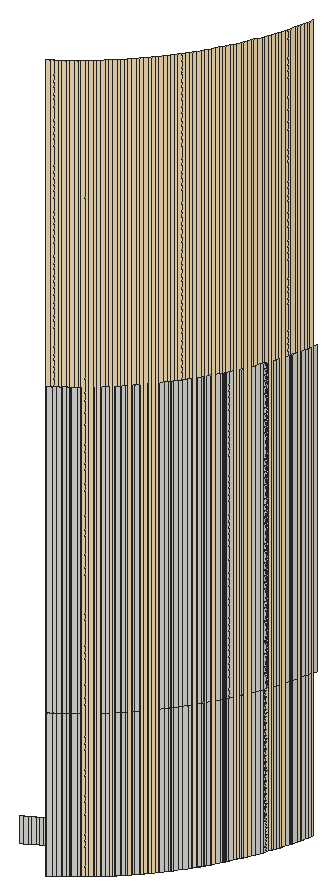
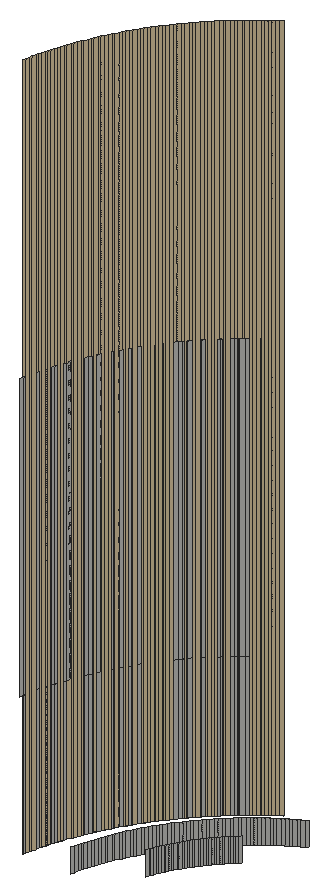
# SketchUp Ruby script. Lengths in inches.
U = 1.inch
M = Sketchup.active_model
def pt(a) = Geom::Point3d.new(a.map { |v| v * U })
def face(e, loops, mat)
  f = e.add_face(loops[0].map { |a| pt(a) })
  loops[1..].each { |l| e.add_face(l.map { |a| pt(a) }).erase! }
  f.material = f.back_material = mat if mat
  f
end
# faces: each face lists its corners as indices into pts; further lists are holes
def faces(e, pts, list, mat = nil) = list.each { |f| face(e, (f[0].is_a?(Array) ? f : [f]).map { |l| l.map { |i| pts[i] } }, mat) }
# xy, xz, yz: faces in a plane at the given z, y or x. An outline is a flat list of corners, or four numbers for a rectangle; further outlines are holes
def ring(l) = l.size == 4 ? [[l[0], l[1]], [l[2], l[1]], [l[2], l[3]], [l[0], l[3]]] : l.each_slice(2).to_a
def flat(e, list, mat, &to3) = list.each { |f| face(e, (f[0].is_a?(Array) ? f : [f]).map { |l| ring(l).map { |u, v| to3.(u, v) } }, mat) }
def xy(e, z, list, mat = nil) = flat(e, list, mat) { |x, y| [x, y, z] }
def xz(e, y, list, mat = nil) = flat(e, list, mat) { |x, z| [x, y, z] }
def yz(e, x, list, mat = nil) = flat(e, list, mat) { |y, z| [x, y, z] }
def lines(e, pts, list) = list.each { |a, b| e.add_line(pt(pts[a]), pt(pts[b])) }
# prism: a flat outline (further loops are holes) pulled along v
def prism(e, loops, v, mat = nil)
  f = face(e, loops, mat); d = Geom::Vector3d.new(v.map { |x| x * U })
  f.pushpull(f.normal.samedirection?(d) ? d.length : -d.length)
end
def box(e, o, s, mat = nil) = prism(e, [[o, [o[0] + s[0], o[1], o[2]], [o[0] + s[0], o[1] + s[1], o[2]], [o[0], o[1] + s[1], o[2]]]], [0, 0, s[2]], mat)
def at(x, y, z, deg = 0) = Geom::Transformation.translation(pt([x, y, z])) * Geom::Transformation.rotation(ORIGIN, Z_AXIS, deg.degrees)
def axes(o, x, y, z) = Geom::Transformation.new([*x, 0, *y, 0, *z, 0, *pt(o).to_a, 1])
def part(name) = M.definitions.add(name)
# library, detail: a bought-in or finely detailed component or shape, given as its bounding box
def library(name, o, s) = part(name).tap { |d| box(d.entities, o, s) }
def detail(e, o, s) = box(e.add_group.entities, o, s)
def put(e, d, t, mat = nil) = e.add_instance(d, t).tap { |i| i.material = mat if mat }
def group(e, t, mat = nil) = e.add_group.tap { |g| g.transformation = t; g.material = mat if mat }.entities
root = M.entities
M.materials.add("1026 AP 7946 SUNNY SIDE UP").color = [254, 231, 186]
p = [[183.75,229.08,246],[183.64,229,246],[183.64,229,276],[183.75,229.08,276],[183.8,229.11,252],[183.67,229.02,252],
  [183.67,229.02,246],[183.8,229.11,246],[183.85,229.15,246],[183.85,229.15,276],[183.95,229.22,246],[183.95,229.22,276],
  [183.93,229.2,252],[183.93,229.2,246],[184.05,229.29,252],[184.05,229.29,246],[184.05,229.29,246],[184.05,229.29,276],
  [184.15,229.37,246],[184.15,229.37,276],[184.18,229.38,252],[184.18,229.38,246],[184.26,229.44,246],[184.26,229.44,276],
  [184.31,229.48,252],[184.31,229.48,246],[184.35,229.52,246],[184.35,229.52,276],[184.43,229.58,252],[184.43,229.58,246],
  [184.45,229.6,246],[184.45,229.6,276],[184.55,229.67,252],[184.55,229.67,246],[184.55,229.67,246],[184.55,229.67,276],
  [184.65,229.75,246],[184.65,229.75,276],[184.67,229.77,252],[184.67,229.77,246],[184.75,229.83,246],[184.75,229.83,276],
  [184.84,229.92,246],[184.84,229.92,276],[184.79,229.875,252],[184.79,229.875,246],[184.9375,230,246],[184.9375,230,276],
  [184.91,229.98,252],[184.91,229.98,246],[185.03,230.08,246],[185.03,230.08,276],[185.03,230.08,252],[185.03,230.08,246],
  [185.12,230.17,246],[185.12,230.17,276],[185.15,230.1875,252],[185.15,230.1875,246],[181.77,230.21,246],[181.66,230.15,246],
  [181.66,230.15,247],[181.77,230.21,247],[181.89,230.28,246],[181.89,230.28,247],[185.21,230.25,246],[185.21,230.25,276],
  [185.26,230.3,252],[185.26,230.3,246],[182,230.34,246],[182,230.34,247],[182.11,230.41,246],[182.11,230.41,247],
  [185.31,230.34,246],[185.31,230.34,276],[185.4,230.43,246],[185.4,230.43,276],[185.375,230.4,252],[185.375,230.4,246],
  [182.22,230.47,246],[182.22,230.47,247],[185.49,230.51,246],[185.49,230.51,276],[185.49,230.51,252],[185.49,230.51,246],
  [182.34,230.54,246],[182.34,230.54,247],[182.45,230.61,246],[182.45,230.61,247],[185.57,230.6,246],[185.57,230.6,276],
  [185.6,230.625,252],[185.6,230.625,246],[182.56,230.69,246],[182.56,230.69,247],[185.66,230.69,246],[185.66,230.69,276],
  [185.7,230.74,252],[185.7,230.74,246],[182.66,230.76,246],[182.66,230.76,247],[185.75,230.79,246],[185.75,230.79,276],
  [185.8125,230.85,252],[185.8125,230.85,246],[182.77,230.83,246],[182.77,230.83,247],[182.88,230.91,246],[182.88,230.91,247],
  [185.83,230.88,246],[185.83,230.88,276],[182.98,230.99,246],[182.98,230.99,247],[185.92,230.97,246],[185.92,230.97,276],
  [185.92,230.97,252],[185.92,230.97,246],[183.09,231.07,246],[183.09,231.07,247],[186,231.0625,246],[186,231.0625,276],
  [186.02,231.09,252],[186.02,231.09,246],[183.19,231.15,246],[183.19,231.15,247],[183.29,231.23,246],[183.29,231.23,247],
  [186.08,231.16,246],[186.08,231.16,276],[186.125,231.21,252],[186.125,231.21,246],[183.39,231.3125,246],[183.39,231.3125,247],
  [186.17,231.25,246],[186.17,231.25,276],[186.23,231.33,252],[186.23,231.33,246],[183.49,231.4,246],[183.49,231.4,247],
  [186.25,231.35,246],[186.25,231.35,276],[186.33,231.45,252],[186.33,231.45,246],[183.59,231.48,246],[183.59,231.48,247],
  [186.33,231.45,246],[186.33,231.45,276],[186.4,231.55,246],[186.4,231.55,276],[186.42,231.57,252],[186.42,231.57,246],
  [183.69,231.57,246],[183.69,231.57,247],[186.48,231.65,246],[186.48,231.65,276],[183.79,231.66,246],[183.79,231.66,247],
  [186.52,231.69,252],[186.52,231.69,246],[186.56,231.74,246],[186.56,231.74,276],[183.88,231.75,246],[183.88,231.75,247],
  [183.98,231.84,246],[183.98,231.84,247],[186.62,231.82,252],[186.62,231.82,246],[186.63,231.85,246],[186.63,231.85,276],
  [184.07,231.93,246],[184.07,231.93,247],[186.71,231.95,246],[186.71,231.95,276],[186.71,231.95,252],[186.71,231.95,246],
  [184.16,232.02,246],[184.16,232.02,247],[186.78,232.05,246],[186.78,232.05,276],[186.8,232.07,252],[186.8,232.07,246],
  [184.25,232.12,246],[184.25,232.12,247],[186.85,232.15,246],[186.85,232.15,276],[184.34,232.21,246],[184.34,232.21,247],
  [186.89,232.2,252],[186.89,232.2,246],[184.43,232.31,246],[184.43,232.31,247],[186.92,232.25,246],[186.92,232.25,276],
  [186.98,232.33,252],[186.98,232.33,246],[184.52,232.41,246],[184.52,232.41,247],[187,232.36,246],[187,232.36,276],
  [187.0625,232.46,252],[187.0625,232.46,246],[184.6,232.51,246],[184.6,232.51,247],[187.0625,232.46,246],[187.0625,232.46,276],
  [184.6875,232.61,246],[184.6875,232.61,247],[187.13,232.57,246],[187.13,232.57,276],[187.15,232.6,252],[187.15,232.6,246],
  [184.77,232.71,246],[184.77,232.71,247],[187.2,232.68,246],[187.2,232.68,276],[187.23,232.73,252],[187.23,232.73,246],
  [184.85,232.81,246],[184.85,232.81,247],[187.26,232.78,246],[187.26,232.78,276],[187.3125,232.86,252],[187.3125,232.86,246],
  [184.93,232.91,246],[184.93,232.91,247],[187.33,232.89,246],[187.33,232.89,276],[185.01,233.02,246],[185.01,233.02,247],
  [187.39,233,246],[187.39,233,276],[187.39,233,252],[187.39,233,246],[185.09,233.12,246],[185.09,233.12,247],
  [187.45,233.11,246],[187.45,233.11,276],[187.47,233.14,252],[187.47,233.14,246],[185.17,233.23,246],[185.17,233.23,247],
  [187.52,233.22,246],[187.52,233.22,276],[187.55,233.27,252],[187.55,233.27,246],[185.24,233.34,246],[185.24,233.34,247],
  [187.58,233.33,246],[187.58,233.33,276],[185.31,233.44,246],[185.31,233.44,247],[187.62,233.41,252],[187.62,233.41,246],
  [187.63,233.44,246],[187.63,233.44,276],[185.39,233.55,246],[185.39,233.55,247],[187.69,233.55,246],[187.69,233.55,276],
  [187.69,233.55,252],[187.69,233.55,246],[185.46,233.66,246],[185.46,233.66,247],[187.75,233.66,246],[187.75,233.66,276],
  [187.76,233.69,252],[187.76,233.69,246],[185.53,233.78,246],[185.53,233.78,247],[187.8,233.78,246],[187.8,233.78,276],
  [187.83,233.83,252],[187.83,233.83,246],[185.59,233.89,246],[185.59,233.89,247],[187.86,233.89,246],[187.86,233.89,276],
  [187.9,233.98,252],[187.9,233.98,246],[185.66,234,246],[185.66,234,247],[187.91,234,246],[187.91,234,276],
  [185.72,234.11,246],[185.72,234.11,247],[187.96,234.12,246],[187.96,234.12,276],[187.96,234.12,252],[187.96,234.12,246],
  [185.79,234.23,246],[185.79,234.23,247],[188.01,234.23,246],[188.01,234.23,276],[188.03,234.26,252],[188.03,234.26,246],
  [185.85,234.34,246],[185.85,234.34,247],[188.0625,234.35,246],[188.0625,234.35,276],[185.91,234.46,246],[185.91,234.46,247],
  [188.09,234.41,252],[188.09,234.41,246],[188.11,234.47,246],[188.11,234.47,276],[188.15,234.55,252],[188.15,234.55,246],
  [185.97,234.58,246],[185.97,234.58,247],[188.16,234.58,246],[188.16,234.58,276],[186.03,234.69,246],[186.03,234.69,247],
  [188.2,234.7,252],[188.2,234.7,246],[188.2,234.7,246],[188.2,234.7,276],[186.08,234.8125,246],[186.08,234.8125,247],
  [188.25,234.82,246],[188.25,234.82,276],[188.26,234.85,252],[188.26,234.85,246],[186.14,234.93,246],[186.14,234.93,247],
  [188.29,234.94,246],[188.29,234.94,276],[188.3125,234.99,252],[188.3125,234.99,246],[186.1875,235.05,246],[186.1875,235.05,247],
  [188.33,235.05,246],[188.33,235.05,276],[188.36,235.14,252],[188.36,235.14,246],[186.24,235.17,246],[186.24,235.17,247],
  [188.375,235.17,246],[188.375,235.17,276],[188.41,235.29,252],[188.41,235.29,246],[186.29,235.29,246],[186.29,235.29,247],
  [188.41,235.29,246],[188.41,235.29,276],[186.34,235.42,246],[186.34,235.42,247],[188.45,235.41,246],[188.45,235.41,276],
  [188.46,235.44,252],[188.46,235.44,246],[186.38,235.54,246],[186.38,235.54,247],[188.49,235.53,246],[188.49,235.53,276],
  [188.51,235.59,252],[188.51,235.59,246],[186.43,235.66,246],[186.43,235.66,247],[188.52,235.65,246],[188.52,235.65,276],
  [188.55,235.74,252],[188.55,235.74,246],[186.47,235.79,246],[186.47,235.79,247],[188.56,235.77,246],[188.56,235.77,276],
  [188.59,235.89,252],[188.59,235.89,246],[186.51,235.91,246],[186.51,235.91,247],[188.59,235.89,246],[188.59,235.89,276],
  [186.55,236.03,246],[186.55,236.03,247],[188.62,236.02,246],[188.62,236.02,276],[188.63,236.05,252],[188.63,236.05,246],
  [186.59,236.16,246],[186.59,236.16,247],[188.65,236.14,246],[188.65,236.14,276],[188.67,236.2,252],[188.67,236.2,246],
  [188.68,236.26,246],[188.68,236.26,276],[186.625,236.29,246],[186.625,236.29,247],[188.7,236.35,252],[188.7,236.35,246],
  [186.66,236.41,246],[186.66,236.41,247],[188.71,236.38,246],[188.71,236.38,276],[181.68,233.8,248],[181.68,233.8,247],
  [181.62,233.74,247],[181.62,233.74,248],[181.75,233.86,248],[181.75,233.86,247],[181.82,233.92,248],[181.82,233.92,247],
  [181.88,233.99,248],[181.88,233.99,247],[181.95,234.05,248],[181.95,234.05,247],[182.01,234.12,248],[182.01,234.12,247],
  [182.08,234.18,248],[182.08,234.18,247],[182.14,234.25,248],[182.14,234.25,247],[182.2,234.32,248],[182.2,234.32,247],
  [182.26,234.38,248],[182.26,234.38,247],[182.32,234.45,248],[182.32,234.45,247],[182.38,234.52,248],[182.38,234.52,247],
  [182.44,234.59,248],[182.44,234.59,247],[182.5,234.67,248],[182.5,234.67,247],[182.55,234.74,248],[182.55,234.74,247],
  [182.61,234.8125,248],[182.61,234.8125,247],[182.66,234.89,248],[182.66,234.89,247],[182.72,234.96,248],[182.72,234.96,247],
  [182.77,235.04,248],[182.77,235.04,247],[182.82,235.11,248],[182.82,235.11,247],[182.87,235.1875,248],[182.87,235.1875,247],
  [182.92,235.26,248],[182.92,235.26,247],[182.97,235.34,248],[182.97,235.34,247],[183.02,235.42,248],[183.02,235.42,247],
  [183.0625,235.5,248],[183.0625,235.5,247],[183.11,235.58,248],[183.11,235.58,247],[183.15,235.66,248],[183.15,235.66,247],
  [183.19,235.74,248],[183.19,235.74,247],[183.24,235.82,248],[183.24,235.82,247],[183.28,235.9,248],[183.28,235.9,247],
  [183.32,235.99,248],[183.32,235.99,247],[183.36,236.07,248],[183.36,236.07,247],[183.39,236.15,248],[183.39,236.15,247],
  [183.43,236.24,248],[183.43,236.24,247],[183.47,236.32,248],[183.47,236.32,247],[183.5,236.41,248],[183.5,236.41,247],
  [183.8,229.11,264],[183.67,229.02,264],[183.67,229.02,252],[183.8,229.11,252],[183.93,229.2,264],[183.93,229.2,252],
  [184.05,229.29,264],[184.05,229.29,252],[184.18,229.38,264],[184.18,229.38,252],[184.31,229.48,264],[184.31,229.48,252],
  [184.43,229.58,264],[184.43,229.58,252],[184.55,229.67,264],[184.55,229.67,252],[184.67,229.77,264],[184.67,229.77,252],
  [184.79,229.875,264],[184.79,229.875,252],[184.91,229.98,264],[184.91,229.98,252],[185.03,230.08,264],[185.03,230.08,252],
  [185.15,230.1875,264],[185.15,230.1875,252],[185.26,230.3,264],[185.26,230.3,252],[185.375,230.4,264],[185.375,230.4,252],
  [185.49,230.51,264],[185.49,230.51,252],[185.6,230.625,264],[185.6,230.625,252],[185.7,230.74,264],[185.7,230.74,252],
  [185.8125,230.85,264],[185.8125,230.85,252],[185.92,230.97,264],[185.92,230.97,252],[186.02,231.09,264],[186.02,231.09,252],
  [186.125,231.21,264],[186.125,231.21,252],[186.23,231.33,264],[186.23,231.33,252],[186.33,231.45,264],[186.33,231.45,252],
  [186.42,231.57,264],[186.42,231.57,252],[186.52,231.69,264],[186.52,231.69,252],[186.62,231.82,264],[186.62,231.82,252],
  [186.71,231.95,264],[186.71,231.95,252],[186.8,232.07,264],[186.8,232.07,252],[186.89,232.2,264],[186.89,232.2,252],
  [186.98,232.33,264],[186.98,232.33,252],[187.0625,232.46,264],[187.0625,232.46,252],[187.15,232.6,264],[187.15,232.6,252],
  [187.23,232.73,264],[187.23,232.73,252],[187.3125,232.86,264],[187.3125,232.86,252],[187.39,233,264],[187.39,233,252],
  [187.47,233.14,264],[187.47,233.14,252],[187.55,233.27,264],[187.55,233.27,252],[187.62,233.41,264],[187.62,233.41,252],
  [187.69,233.55,264],[187.69,233.55,252],[187.76,233.69,264],[187.76,233.69,252],[187.83,233.83,264],[187.83,233.83,252],
  [187.9,233.98,264],[187.9,233.98,252],[187.96,234.12,264],[187.96,234.12,252],[188.03,234.26,264],[188.03,234.26,252],
  [188.09,234.41,264],[188.09,234.41,252],[188.15,234.55,264],[188.15,234.55,252],[188.2,234.7,264],[188.2,234.7,252],
  [188.26,234.85,264],[188.26,234.85,252],[188.3125,234.99,264],[188.3125,234.99,252],[188.36,235.14,264],[188.36,235.14,252],
  [188.41,235.29,264],[188.41,235.29,252],[188.46,235.44,264],[188.46,235.44,252],[188.51,235.59,264],[188.51,235.59,252],
  [188.55,235.74,264],[188.55,235.74,252],[188.59,235.89,264],[188.59,235.89,252],[188.63,236.05,264],[188.63,236.05,252],
  [188.67,236.2,264],[188.67,236.2,252],[188.7,236.35,264],[188.7,236.35,252],[188.74,236.51,264],[188.74,236.51,252],
  [186.61,236.43,246],[186.57,236.3,246],[186.54,236.18,246],[186.5,236.05,246],[186.46,235.93,246],[186.42,235.8,246],
  [186.375,235.68,246],[186.33,235.56,246],[186.28,235.4375,246],[186.24,235.31,246],[186.1875,235.19,246],[186.14,235.07,246],
  [186.09,234.95,246],[186.03,234.84,246],[185.98,234.72,246],[185.92,234.6,246],[185.86,234.48,246],[185.8,234.37,246],
  [185.74,234.25,246],[185.68,234.14,246],[185.61,234.03,246],[185.55,233.92,246],[185.48,233.8,246],[185.41,233.69,246],
  [185.34,233.58,246],[185.27,233.47,246],[185.2,233.37,246],[185.12,233.26,246],[185.05,233.15,246],[184.97,233.05,246],
  [184.89,232.95,246],[184.81,232.84,246],[184.73,232.74,246],[184.65,232.64,246],[184.5625,232.54,246],[184.48,232.44,246],
  [184.39,232.35,246],[184.3,232.25,246],[184.21,232.15,246],[184.125,232.06,246],[184.03,231.97,246],[183.94,231.875,246],
  [183.85,231.79,246],[183.75,231.7,246],[183.65,231.61,246],[183.56,231.52,246],[183.46,231.4375,246],[183.36,231.35,246],
  [183.26,231.27,246],[183.16,231.19,246],[183.05,231.11,246],[182.95,231.03,246],[182.85,230.95,246],[182.74,230.88,246],
  [182.63,230.8,246],[182.53,230.73,246],[182.42,230.66,246],[182.31,230.59,246],[182.2,230.52,246],[182.08,230.45,246],
  [181.97,230.39,246],[181.86,230.32,246],[181.75,230.26,246],[181.63,230.2,246]]
faces(root,p,[[0,1,2,3],[8,0,3,9],[10,8,9,11],[16,10,11,17],[18,16,17,19],[22,18,19,23],[26,22,23,27],[30,26,27,31],
  [34,30,31,35],[36,34,35,37],[40,36,37,41],[42,40,41,43],[46,42,43,47],[50,46,47,51],[54,50,51,55],[64,54,55,65],
  [72,64,65,73],[74,72,73,75],[80,74,75,81],[88,80,81,89],[94,88,89,95],[100,94,95,101],[108,100,101,109],[112,108,109,113],
  [118,112,113,119],[126,118,119,127],[132,126,127,133],[138,132,133,139],[144,138,139,145],[146,144,145,147],[152,146,147,153],[158,152,153,159],
  [166,158,159,167],[170,166,167,171],[176,170,171,177],[182,176,177,183],[190,182,183,191],[196,190,191,197],[202,196,197,203],[206,202,203,207],
  [212,206,207,213],[218,212,213,219],[224,218,219,225],[228,224,225,229],[234,228,229,235],[240,234,235,241],[246,240,241,247],[252,246,247,253],
  [256,252,253,257],[262,256,257,263],[268,262,263,269],[274,268,269,275],[280,274,275,281],[284,280,281,285],[290,284,285,291],[296,290,291,297],
  [302,296,297,303],[308,302,303,309],[314,308,309,315],[318,314,315,319],[324,318,319,325],[330,324,325,331],[336,330,331,337],[342,336,337,343],
  [346,342,343,347],[352,346,347,353],[358,352,353,359],[364,358,359,365],[370,364,365,371],[374,370,371,375],[380,374,375,381],[384,380,381,385],
  [392,384,385,393]],"1026 AP 7946 SUNNY SIDE UP")
faces(root,p,[[4,5,6,7],[12,4,7,13],[14,12,13,15],[20,14,15,21],[24,20,21,25],[28,24,25,29],[32,28,29,33],[38,32,33,39],
  [44,38,39,45],[48,44,45,49],[52,48,49,53],[56,52,53,57],[58,59,60,61],[62,58,61,63],[66,56,57,67],[68,62,63,69],
  [70,68,69,71],[76,66,67,77],[78,70,71,79],[82,76,77,83],[84,78,79,85],[86,84,85,87],[90,82,83,91],[92,86,87,93],
  [96,90,91,97],[98,92,93,99],[102,96,97,103],[104,98,99,105],[106,104,105,107],[110,106,107,111],[114,102,103,115],[116,110,111,117],
  [120,114,115,121],[122,116,117,123],[124,122,123,125],[128,120,121,129],[130,124,125,131],[134,128,129,135],[136,130,131,137],[140,134,135,141],
  [142,136,137,143],[148,140,141,149],[150,142,143,151],[154,150,151,155],[156,148,149,157],[160,154,155,161],[162,160,161,163],[164,156,157,165],
  [168,162,163,169],[172,164,165,173],[174,168,169,175],[178,172,173,179],[180,174,175,181],[184,180,181,185],[186,178,179,187],[188,184,185,189],
  [192,186,187,193],[194,188,189,195],[198,192,193,199],[200,194,195,201],[204,200,201,205],[208,198,199,209],[210,204,205,211],[214,208,209,215],
  [216,210,211,217],[220,214,215,221],[222,216,217,223],[226,222,223,227],[230,220,221,231],[232,226,227,233],[236,230,231,237],[238,232,233,239],
  [242,236,237,243],[244,238,239,245],[248,244,245,249],[250,242,243,251],[254,248,249,255],[258,250,251,259],[260,254,255,261],[264,258,259,265],
  [266,260,261,267],[270,264,265,271],[272,266,267,273],[276,270,271,277],[278,272,273,279],[282,278,279,283],[286,276,277,287],[288,282,283,289],
  [292,286,287,293],[294,288,289,295],[298,294,295,299],[300,292,293,301],[304,300,301,305],[306,298,299,307],[310,306,307,311],[312,304,305,313],
  [316,310,311,317],[320,312,313,321],[322,316,317,323],[326,320,321,327],[328,322,323,329],[332,326,327,333],[334,328,329,335],[338,332,333,339],
  [340,334,335,341],[344,340,341,345],[348,338,339,349],[350,344,345,351],[354,348,349,355],[356,350,351,357],[360,354,355,361],[362,356,357,363],
  [366,360,361,367],[368,362,363,369],[372,368,369,373],[376,366,367,377],[378,372,373,379],[382,376,377,383],[386,378,379,387],[388,382,383,389],
  [390,386,387,391],[394,395,396,397],[398,399,395,394],[400,401,399,398],[402,403,401,400],[404,405,403,402],[406,407,405,404],[408,409,407,406],
  [410,411,409,408],[412,413,411,410],[414,415,413,412],[416,417,415,414],[418,419,417,416],[420,421,419,418],[422,423,421,420],[424,425,423,422],
  [426,427,425,424],[428,429,427,426],[430,431,429,428],[432,433,431,430],[434,435,433,432],[436,437,435,434],[438,439,437,436],[440,441,439,438],
  [442,443,441,440],[444,445,443,442],[446,447,445,444],[448,449,447,446],[450,451,449,448],[452,453,451,450],[454,455,453,452],[456,457,455,454],
  [458,459,457,456],[460,461,459,458],[462,463,461,460],[464,465,463,462],[466,467,465,464],[468,469,470,471],[472,468,471,473],[474,472,473,475],
  [476,474,475,477],[478,476,477,479],[480,478,479,481],[482,480,481,483],[484,482,483,485],[486,484,485,487],[488,486,487,489],[490,488,489,491],
  [492,490,491,493],[494,492,493,495],[496,494,495,497],[498,496,497,499],[500,498,499,501],[502,500,501,503],[504,502,503,505],[506,504,505,507],
  [508,506,507,509],[510,508,509,511],[512,510,511,513],[514,512,513,515],[516,514,515,517],[518,516,517,519],[520,518,519,521],[522,520,521,523],
  [524,522,523,525],[526,524,525,527],[528,526,527,529],[530,528,529,531],[532,530,531,533],[534,532,533,535],[536,534,535,537],[538,536,537,539],
  [540,538,539,541],[542,540,541,543],[544,542,543,545],[546,544,545,547],[548,546,547,549],[550,548,549,551],[552,550,551,553],[554,552,553,555],
  [556,554,555,557],[558,556,557,559],[560,558,559,561],[562,560,561,563],[564,562,563,565],[566,564,565,567],[568,566,567,569],[570,568,569,571],
  [572,570,571,573],[574,572,573,575],[576,574,575,577],[578,576,577,579],[580,578,579,581],[582,580,581,583],[584,582,583,585],[586,584,585,587]])
lines(root,p,[[588,589],[589,590],[590,591],[591,592],[592,593],[593,594],[594,595],[595,596],[596,597],[597,598],[598,599],[599,600],
  [600,601],[601,602],[602,603],[603,604],[604,605],[605,606],[606,607],[607,608],[608,609],[609,610],[610,611],[611,612],
  [612,613],[613,614],[614,615],[615,616],[616,617],[617,618],[618,619],[619,620],[620,621],[621,622],[622,623],[623,624],
  [624,625],[625,626],[626,627],[627,628],[628,629],[629,630],[630,631],[631,632],[632,633],[633,634],[634,635],[635,636],
  [636,637],[637,638],[638,639],[639,640],[640,641],[641,642],[642,643],[643,644],[644,645],[645,646],[646,647],[647,648],
  [648,649],[649,650],[650,651]])
